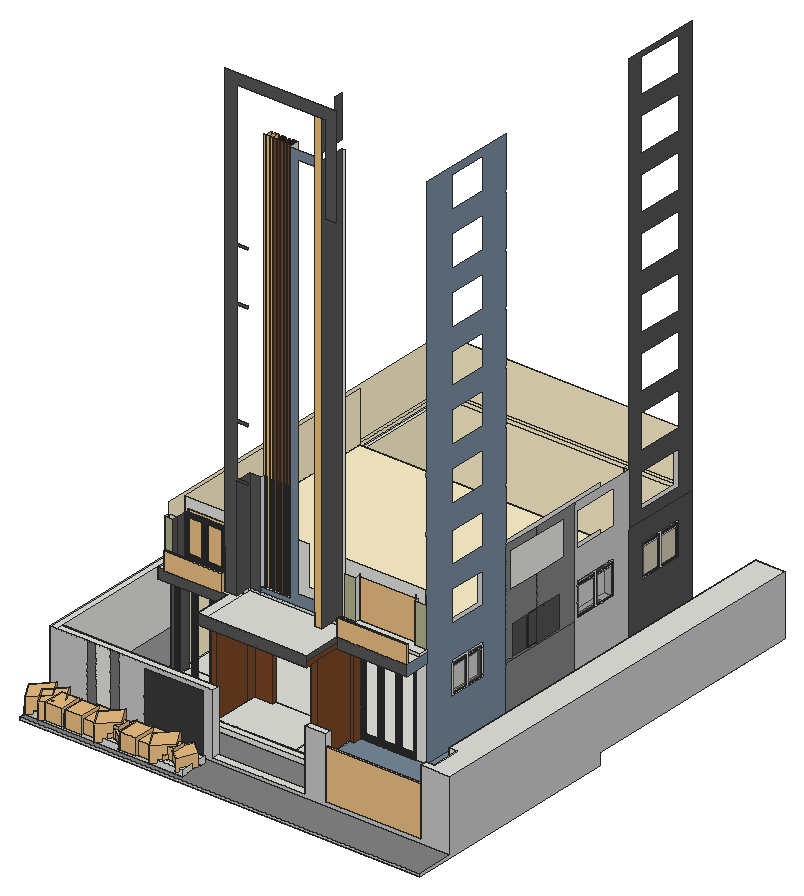
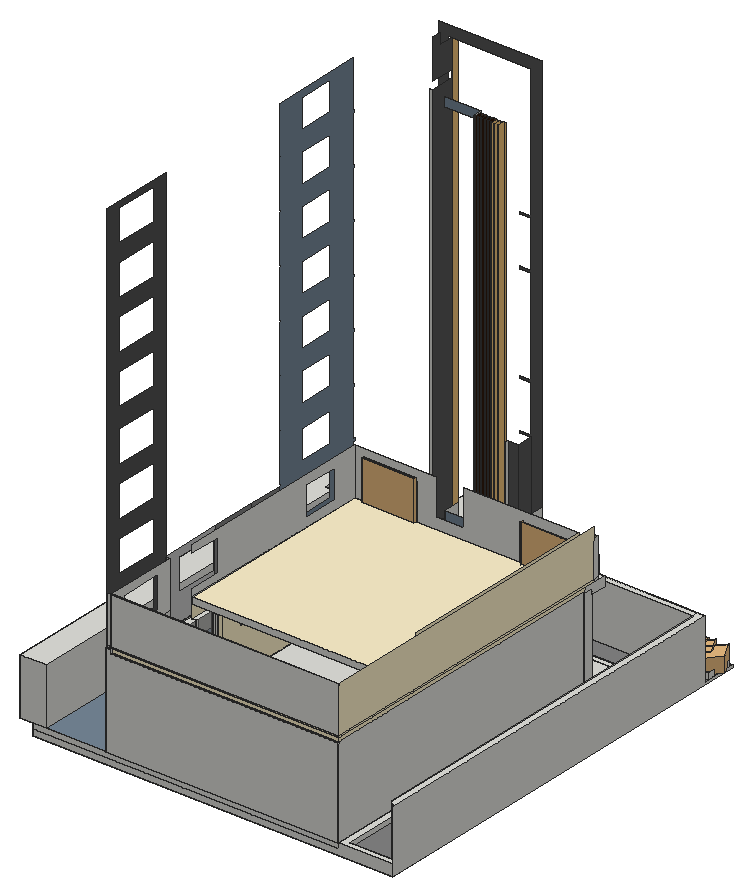
# SketchUp Ruby script. Lengths in inches.
U = 1.inch
M = Sketchup.active_model
def pt(a) = Geom::Point3d.new(a.map { |v| v * U })
def face(e, loops, mat)
  f = e.add_face(loops[0].map { |a| pt(a) })
  loops[1..].each { |l| e.add_face(l.map { |a| pt(a) }).erase! }
  f.material = f.back_material = mat if mat
  f
end
# faces: each face lists its corners as indices into pts; further lists are holes
def faces(e, pts, list, mat = nil) = list.each { |f| face(e, (f[0].is_a?(Array) ? f : [f]).map { |l| l.map { |i| pts[i] } }, mat) }
# xy, xz, yz: faces in a plane at the given z, y or x. An outline is a flat list of corners, or four numbers for a rectangle; further outlines are holes
def ring(l) = l.size == 4 ? [[l[0], l[1]], [l[2], l[1]], [l[2], l[3]], [l[0], l[3]]] : l.each_slice(2).to_a
def flat(e, list, mat, &to3) = list.each { |f| face(e, (f[0].is_a?(Array) ? f : [f]).map { |l| ring(l).map { |u, v| to3.(u, v) } }, mat) }
def xy(e, z, list, mat = nil) = flat(e, list, mat) { |x, y| [x, y, z] }
def xz(e, y, list, mat = nil) = flat(e, list, mat) { |x, z| [x, y, z] }
def yz(e, x, list, mat = nil) = flat(e, list, mat) { |y, z| [x, y, z] }
def lines(e, pts, list) = list.each { |a, b| e.add_line(pt(pts[a]), pt(pts[b])) }
# prism: a flat outline (further loops are holes) pulled along v
def prism(e, loops, v, mat = nil)
  f = face(e, loops, mat); d = Geom::Vector3d.new(v.map { |x| x * U })
  f.pushpull(f.normal.samedirection?(d) ? d.length : -d.length)
end
def box(e, o, s, mat = nil) = prism(e, [[o, [o[0] + s[0], o[1], o[2]], [o[0] + s[0], o[1] + s[1], o[2]], [o[0], o[1] + s[1], o[2]]]], [0, 0, s[2]], mat)
def at(x, y, z, deg = 0) = Geom::Transformation.translation(pt([x, y, z])) * Geom::Transformation.rotation(ORIGIN, Z_AXIS, deg.degrees)
def axes(o, x, y, z) = Geom::Transformation.new([*x, 0, *y, 0, *z, 0, *pt(o).to_a, 1])
def part(name) = M.definitions.add(name)
# library, detail: a bought-in or finely detailed component or shape, given as its bounding box
def library(name, o, s) = part(name).tap { |d| box(d.entities, o, s) }
def detail(e, o, s) = box(e.add_group.entities, o, s)
def put(e, d, t, mat = nil) = e.add_instance(d, t).tap { |i| i.material = mat if mat }
def group(e, t, mat = nil) = e.add_group.tap { |g| g.transformation = t; g.material = mat if mat }.entities
root = M.entities
M.materials.add("Material__1").color = [95, 70, 46]
M.materials.add("Wine2").color = [0, 0, 0]
M.materials["Wine2"].alpha = 0
M.materials.add("[0110_LightSlateGray]").color = [119, 136, 153]
M.materials.add("[0130_Gainsboro]").color = [39, 45, 50]
M.materials.add("[0133_Gray]").color = [128, 128, 128]
M.materials.add("[0135_DarkGray]1").color = [81, 81, 81]
M.materials.add("[Color D01]").color = [255, 242, 204]
M.materials.add("[Color E01]").color = [178, 178, 142]
M.materials.add("[Color M02]").color = [198, 198, 198]
M.materials.add("[Color M05]").color = [114, 114, 114]
M.materials.add("[Color M06]").color = [86, 86, 86]
M.materials.add("[Color M07]").color = [58, 58, 58]
M.materials.add("[Tile Grey]").color = [132, 132, 132]
M.materials.add("[Translucent Glass Gray]").color = [128, 128, 128]
M.materials["[Translucent Glass Gray]"].alpha = 0.5
M.materials.add("[Wood Bamboo]").color = [214, 127, 52]
M.materials.add("[Wood Cherry Original]").color = [48, 27, 13]
M.materials.add("[Wood OSB]").color = [240, 195, 122]
M.materials.add("[Wood Veneer 01]").color = [120, 70, 37]
c1 = library("Group\#74",[-84.69,-90.07,-0.36],[176.51,175.13,171.4])
c2 = library("Areca palm plant",[0,0,0],[49.1,36.6,54.46])
c3 = library("Group\#130",[-7.34,-1.2,0],[38.67,35.81,49.04])
c4 = library("Group20\#1",[-20.81,-17.08,3.79],[39.86,39.43,37.51])
c5 = library("Group38\#2",[14.01,28.44,-23.43],[18.58,18.32,38.89])
c6 = library("Slatted entrance gates",[-0.09,68.76,-0.1],[160,5.32,60.06])
c7 = part("Framed glazing panel")
xy(c7.entities,0,[[0,-0.98,43.07,0],[0,0,43.07,1.4]],"[0130_Gainsboro]")
xy(c7.entities,0.3,[[0.3,-1.43,42.77,-0.98]],"[0130_Gainsboro]")
xy(c7.entities,2.95,[[2.95,-1.43,40.12,-0.63],[2.95,-0.63,40.12,0],[2.95,0,40.12,0.64],[2.95,0.64,40.12,1.4]],"[0130_Gainsboro]")
xy(c7.entities,3.54,[[3.54,-0.63,39.53,0],[3.54,0,39.53,0.64]],"[0130_Gainsboro]")
xy(c7.entities,111.8125,[[3.54,-0.63,39.53,0],[3.54,0,39.53,0.64]],"[0130_Gainsboro]")
xy(c7.entities,112.4,[[2.95,-1.43,40.12,-0.63],[2.95,-0.63,40.12,0],[2.95,0,40.12,0.64],[2.95,0.64,40.12,1.4]],"[0130_Gainsboro]")
xy(c7.entities,115.05,[[0.3,-1.43,42.77,-0.98]],"[0130_Gainsboro]")
xy(c7.entities,115.35,[[0,-0.98,43.07,0],[0,0,43.07,1.4]],"[0130_Gainsboro]")
xz(c7.entities,-1.43,[[[0.3,0.3,42.77,115.05],[2.95,2.95,40.12,112.4]]],"[0130_Gainsboro]")
xz(c7.entities,-0.98,[[[0,0,43.07,115.35],[0.3,0.3,42.77,115.05]]],"[0130_Gainsboro]")
xz(c7.entities,-0.63,[[[2.95,2.95,40.12,112.4],[3.54,3.54,39.53,111.8125]]],"[0130_Gainsboro]")
xz(c7.entities,0,[[3.54,3.54,39.53,111.8125]],"Wine2")
xz(c7.entities,0,[[[0,0,43.07,115.35],[2.95,2.95,40.12,112.4]],[[2.95,2.95,40.12,112.4],[3.54,3.54,39.53,111.8125]]],"[0130_Gainsboro]")
xz(c7.entities,0.64,[[[2.95,2.95,40.12,112.4],[3.54,3.54,39.53,111.8125]]],"[0130_Gainsboro]")
xz(c7.entities,1.4,[[[0,0,43.07,115.35],[2.95,2.95,40.12,112.4]]],"[0130_Gainsboro]")
yz(c7.entities,0,[[-0.98,0,0,115.35],[0,0,1.4,115.35]],"[0130_Gainsboro]")
yz(c7.entities,0.3,[[-1.43,0.3,-0.98,115.05]],"[0130_Gainsboro]")
yz(c7.entities,2.95,[[-1.43,2.95,-0.63,112.4],[-0.63,2.95,0,112.4],[0,2.95,0.64,112.4],[0.64,2.95,1.4,112.4]],"[0130_Gainsboro]")
yz(c7.entities,3.54,[[-0.63,3.54,0,111.8125],[0,3.54,0.64,111.8125]],"[0130_Gainsboro]")
yz(c7.entities,39.53,[[-0.63,3.54,0,111.8125],[0,3.54,0.64,111.8125]],"[0130_Gainsboro]")
yz(c7.entities,40.12,[[-1.43,2.95,-0.63,112.4],[-0.63,2.95,0,112.4],[0,2.95,0.64,112.4],[0.64,2.95,1.4,112.4]],"[0130_Gainsboro]")
yz(c7.entities,42.77,[[-1.43,0.3,-0.98,115.05]],"[0130_Gainsboro]")
yz(c7.entities,43.07,[[-0.98,0,0,115.35],[0,0,1.4,115.35]],"[0130_Gainsboro]")
c8 = part("Glazing assembly")
put(c8.entities,c7,axes([90.57,1.43,0],[1.05148,0,0],[0,1,0],[0,0,1]))
put(c8.entities,c7,axes([0,1.43,0],[1.05148,0,0],[0,1,0],[0,0,1]))
put(c8.entities,c7,axes([45.29,1.43,0],[1.05148,0,0],[0,1,0],[0,0,1]))
c9 = part("Group\#3")
xy(c9.entities,0,[[0,0,32.48,1.97]])
xy(c9.entities,0.98,[[0.98,0,31.5,0.98],[0.98,0.98,31.5,1.97]])
xy(c9.entities,8.86,[[0.98,0,31.5,0.98],[0.98,0.98,31.5,1.97]])
xy(c9.entities,9.84,[[0,0,32.48,1.97]])
xz(c9.entities,0,[[[0,0,32.48,9.84],[0.98,0.98,31.5,8.86]]])
xz(c9.entities,0.98,[[0.98,0.98,31.5,8.86]],"[Translucent Glass Gray]")
xz(c9.entities,1.97,[[[0,0,32.48,9.84],[0.98,0.98,31.5,8.86]]])
yz(c9.entities,0,[[0,0,1.97,9.84]])
yz(c9.entities,0.98,[[0,0.98,0.98,8.86],[0.98,0.98,1.97,8.86]])
yz(c9.entities,31.5,[[0,0.98,0.98,8.86],[0.98,0.98,1.97,8.86]])
yz(c9.entities,32.48,[[0,0,1.97,9.84]])
c10 = part("Group\#4")
xy(c10.entities,0,[[0,0,32.48,1.97]])
xy(c10.entities,0.98,[[0.98,0,31.5,0.98],[0.98,0.98,31.5,1.97]])
xy(c10.entities,71.85,[[0.98,0,31.5,0.98],[0.98,0.98,31.5,1.97]])
xy(c10.entities,72.83,[[0,0,32.48,1.97]])
xz(c10.entities,0,[[[0,0,32.48,72.83],[0.98,0.98,31.5,71.85]]])
xz(c10.entities,0.98,[[0.98,0.98,31.5,71.85]],"[Translucent Glass Gray]")
xz(c10.entities,1.97,[[[0,0,32.48,72.83],[0.98,0.98,31.5,71.85]]])
yz(c10.entities,0,[[0,0,1.97,72.83]])
yz(c10.entities,0.98,[[0,0.98,0.98,71.85],[0.98,0.98,1.97,71.85]])
yz(c10.entities,31.5,[[0,0.98,0.98,71.85],[0.98,0.98,1.97,71.85]])
yz(c10.entities,32.48,[[0,0,1.97,72.83]])
c11 = part("FIXED+GLASS+WINDOW+WITH+TRANSOM")
g1 = group(c11.entities,at(0,0,0))
xy(g1,0,[[0,0,70.86,3.9375]])
xy(g1,1.97,[[1.97,0,34.45,0.98],[36.42,0,68.9,3.9375],[1.97,2.95,34.45,3.9375]])
xy(g1,86.61,[[1.97,0,34.45,3.9375],[34.45,0,36.42,3.9375],[36.42,0,68.9,3.9375]])
xy(g1,88.58,[[0,0,70.86,3.9375]])
xz(g1,0,[[[0,0,70.86,88.58],[1.97,1.97,34.45,86.61],[36.42,1.97,68.9,86.61]]])
xz(g1,3.9375,[[[0,0,70.86,88.58],[1.97,1.97,34.45,86.61],[36.42,1.97,68.9,86.61]]])
yz(g1,0,[[0,0,3.9375,88.58]])
yz(g1,1.97,[[0,1.97,3.9375,74.8],[0,76.77,3.9375,86.61]])
yz(g1,34.45,[[0,1.97,3.9375,86.61]])
yz(g1,36.42,[[0,1.97,3.9375,86.61]])
yz(g1,68.9,[[0,1.97,3.9375,86.61]])
yz(g1,70.86,[[0,0,3.9375,88.58]])
g2 = group(g1,at(1.97,0,74.8))
box(g2,[0,0,0],[66.93,3.9375,1.97])
put(g1,c9,at(1.97,0.98,76.77))
put(g1,c9,at(36.42,0.98,76.77))
put(g1,c10,at(1.97,0.98,1.97))
put(g1,c10,at(36.42,0.98,1.97))
c12 = library("Glass Railing",[0,0,0],[139.5,4.76,42])
c13 = library("Group5_1",[-7.56,-66.38,0.11],[6.33,135.04,120.95])
xy(root,-23.6875,[[0,0,0,1091.875,923.0625,1091.875,923.0625,537.75,956.9375,537.75,956.9375,0]])
xy(root,-17.4,[[0,0,956.9375,91]],"[Tile Grey]")
xy(root,-8,[[389.92,91,609.52,107.02],[658.23,91,886.57,107.02]])
xy(root,-8,[[16.02,107.02,907.04,107.02,907.04,173.85,121.35,173.85,121.35,1075.85,16.02,1075.85]],"[Tile Grey]")
xy(root,4.3125,[[121.35,173.85,886.57,173.85,886.57,189.875,137.375,189.875,137.375,1091.875,0,1091.875,16.02,1075.85,121.35,1075.85],[156.37,189.875,304.43,310.82],[363.41,189.875,507.41,310.82],[565.09,189.875,706.35,310.82]])
xy(root,5.625,[[547.97,185.5625,565.09,189.875],[137.375,189.875,156.37,280.75],[156.37,189.875,304.43,310.82],[304.43,189.875,304.43,310.82,363.41,310.82,363.41,301.625,320.43,301.625,320.43,189.875],[320.43,189.875,507.41,189.875,507.41,310.82,363.41,310.82,363.41,301.625,320.43,301.625],
  [507.41,189.875,547.97,301.625],[547.97,189.875,547.97,301.625,507.41,301.625,507.41,310.82,565.09,310.82,565.09,189.875],[565.09,279.375,575.47,310.82],[137.375,280.75,156.37,310.82],[706.35,301.625,733.4375,301.625,733.4375,1091.875,146.57,1091.875,146.57,832.49,721.74,832.49,721.74,310.82,706.35,310.82],
  [137.375,310.82,146.57,1091.875],[146.57,310.82,721.74,832.49],[733.4375,904.3,733.625,1091.875],[137.375,1091.875,733.4375,1094.4375]])
xy(root,5.625,[[565.09,189.875,886.57,189.875,886.57,1091.875,733.625,1091.875,733.625,904.3,733.4375,904.3,733.4375,301.625,706.35,301.625,706.35,310.82,575.47,310.82,575.47,279.375,565.09,279.375]],"[0110_LightSlateGray]")
xy(root,5.625,[[923.0625,537.75,956.9375,744.22],[923.0625,744.22,956.9375,904.3],[923.0625,904.3,956.9375,1091.875]],"[Color M02]")
xy(root,119.72,[[721.74,375.23,733.4375,467.6]])
xy(root,120.06,[[719.43,538.27,721.74,678.14]])
xy(root,120.52,[[711.11,750.25,721.74,832.49],[721.74,750.25,733.4375,750.25,733.4375,861.32,711.11,861.32,711.11,832.49,721.74,832.49],[733.4375,942.08,733.625,1053.14]])
xy(root,137,[[0,91,16.02,91,16.02,1075.85,0,1091.875],[16.02,91,389.92,107.02],[609.52,91,658.23,107.02]])
xy(root,150.625,[[886.57,91,956.9375,91,956.9375,1091.875,886.57,1091.875,886.57,173.85,907.04,173.85,907.04,107.02,886.57,107.02]])
xy(root,194.22,[[721.74,375.23,733.4375,467.6]])
xy(root,201.77,[[711.11,750.25,721.74,832.49],[721.74,750.25,721.74,832.49,711.11,832.49,711.11,861.32,733.4375,861.32,733.4375,750.25],[733.4375,942.08,733.625,1053.14]])
xy(root,202.93,[[719.43,538.27,721.74,678.14]])
xy(root,205.15,[[363.41,301.625,507.41,310.82]])
xy(root,220.35,[[304.43,151.125,304.43,189.875,320.43,189.875,320.43,279.375,547.97,279.375,547.97,185.5625,565.09,185.5625,565.09,151.125],[320.43,279.375,547.97,301.625]],"[Wood Bamboo]")
xy(root,220.77,[[137.375,240.3125,137.375,280.75,156.37,280.75,156.37,301.625,304.43,301.625,304.43,240.3125],[565.09,240.3125,565.09,279.375,575.47,279.375,575.47,301.625,733.4375,301.625,733.4375,240.3125]],"[Wood Bamboo]")
xy(root,233.58,[[156.37,301.625,304.43,310.82]])
xy(root,234.19,[[575.47,301.625,706.35,310.82]])
xy(root,236.5,[[137.375,310.82,146.57,1091.875],[137.375,1091.875,721.74,1094.4375]])
xy(root,245.625,[[304.43,151.125,326.68,261.5],[326.68,151.125,565.09,279.375],[137.375,240.3125,304.43,261.5],[565.09,240.3125,733.4375,279.375],[137.375,261.5,304.43,273.3125],
  [304.43,261.5,326.68,273.3125],[304.43,273.3125,326.68,279.375],[733.4375,904.3,733.625,1091.875],[721.74,1091.875,733.4375,1094.4375]])
xy(root,251.625,[[298.7,240.0625,326.68,261.5],[514.85,240.0625,529.32,279.375],[137.375,261.5,157.82,273.3125],[157.82,261.5,298.7,273.3125],[298.7,261.5,326.68,273.3125],
  [157.82,273.3125,298.7,310.82],[298.7,273.3125,298.7,310.82,563.32,310.82,563.32,301.625,529.32,301.625,529.32,279.375,326.68,279.375,326.68,273.3125],[529.32,279.375,536.21,301.625],[536.21,279.375,563.32,301.625],[563.32,279.375,563.32,310.82,704.2,310.82,704.2,301.625,733.4375,301.625,733.4375,279.375],
  [137.375,1091.875,721.74,1092.875]])
xy(root,251.625,[[146.57,310.82,721.74,832.49]],"[Color D01]")
xy(root,262.54,[[354.04,279.375,423.66,279.375,423.66,301.625,419.15,301.625,419.15,285.875,413.1,285.875,413.1,301.625,410.71,301.625,410.71,285.875,404.66,285.875,404.66,301.625,402.28,301.625,402.28,285.875,396.22,285.875,396.22,301.625,393.84,301.625,393.84,285.875,387.79,285.875,387.79,301.625,385.4,301.625,385.4,285.875,379.35,285.875,379.35,301.625,376.96,301.625,376.96,285.875,370.91,285.875,370.91,301.625,368.53,301.625,368.53,285.875,362.47,285.875,362.47,301.625,360.09,301.625,360.09,285.875,354.04,285.875]])
xz(root,0,[[0,-23.6875,956.9375,-17.4]],"[Color M02]")
xz(root,91,[[107.87,-17.4,141.375,137]])
xz(root,91,[[0,-17.4,87.26,137],[162.87,-17.4,223.1,-17.4,223.1,126.22,366.73,126.22,366.73,-17.4,956.9375,-17.4,956.9375,150.625,886.57,150.625,886.57,-8,658.23,-8,658.23,137,609.52,137,609.52,-8,389.92,-8,389.92,137,162.87,137]],"[Color M02]")
xz(root,91,[[87.26,-17.4,107.87,137],[141.375,-17.4,162.87,137]],"[Color M05]")
xz(root,91,[[223.1,-17.4,366.73,126.22]],"[Color M07]")
xz(root,107.02,[[16.02,-8,389.92,137],[609.52,-8,658.23,137],[886.57,-8,907.04,150.625]])
xz(root,151.125,[[304.43,220.35,565.09,245.625]],"[Color M06]")
xz(root,173.85,[[121.35,-8,156.37,4.3125],[156.37,-8,886.57,4.3125],[886.57,-8,907.04,150.625]])
xz(root,185.5625,[[547.97,5.625,565.09,220.35]],"[Wood Veneer 01]")
xz(root,189.875,[[137.375,4.3125,156.37,5.625],[156.37,4.3125,304.43,5.625],[304.43,4.3125,363.41,5.625],[363.41,4.3125,507.41,5.625],[507.41,4.3125,565.09,5.625],
  [565.09,4.3125,706.35,5.625],[706.35,4.3125,886.57,5.625]])
xz(root,189.875,[[304.43,5.625,320.43,220.35]],"[Wood Veneer 01]")
xz(root,240.0625,[[298.7,251.625,326.68,251.625,326.68,497.625,354.04,497.625,354.04,503.625,326.68,503.625,326.68,623.625,354.04,623.625,354.04,629.625,326.68,629.625,326.68,875.625,354.04,875.625,354.04,881.625,326.68,881.625,326.68,1001.625,354.04,1001.625,354.04,1007.625,326.68,1007.625,326.68,1345.48,539.29,1345.48,539.29,1133.625,563.32,1133.625,563.32,1373.625,298.7,1373.625]],"[Color M06]")
xz(root,240.0625,[[514.85,251.625,529.32,1345.48]],"[Wood OSB]")
xz(root,240.3125,[[137.375,220.77,304.43,245.625],[565.09,220.77,733.4375,245.625]],"[Color M06]")
xz(root,261.5,[[137.375,245.625,326.68,251.625]])
xz(root,261.5,[[137.375,251.625,157.82,345.6875]],"[Color E01]")
xz(root,273.3125,[[137.375,245.625,326.68,251.625],[137.375,251.625,157.82,345.6875]])
xz(root,279.375,[[326.68,245.625,354.04,251.625],[354.04,245.625,733.4375,251.625]])
xz(root,279.375,[[354.04,251.625,514.85,251.625,514.85,279.6,442.42,279.6,442.42,1208.73,514.85,1208.73,514.85,1230.97,423.66,1230.97,423.66,262.54,354.04,262.54]],"[0110_LightSlateGray]")
xz(root,279.375,[[326.68,251.625,354.04,497.625]],"[Color M06]")
xz(root,279.375,[[565.09,5.625,575.47,220.77]],"[Wood Veneer 01]")
xz(root,280.75,[[137.375,5.625,156.37,220.77]],"[Color M06]")
xz(root,285.875,[[354.04,262.54,360.09,1230.97],[362.47,262.54,368.53,1230.97],[370.91,262.54,376.96,1230.97]],"[Wood OSB]")
xz(root,285.875,[[379.35,262.54,385.4,1230.97],[387.79,262.54,393.84,1230.97],[396.22,262.54,402.28,1230.97],[404.66,262.54,410.71,1230.97],[413.1,262.54,419.15,1230.97]],"[Wood Veneer 01]")
xz(root,301.625,[[706.35,5.625,733.4375,220.77],[156.37,220.77,304.43,233.58],[575.47,220.77,706.35,234.19],[704.2,236.5,733.4375,245.625],[704.2,245.625,733.4375,251.625],
  [529.32,251.625,536.21,1253.625],[360.09,262.54,362.47,1230.97],[368.53,262.54,370.91,1230.97],[376.96,262.54,379.35,1230.97]])
xz(root,301.625,[[536.21,251.625,563.32,345.6875],[704.2,251.625,733.4375,345.6875]],"[Color E01]")
xz(root,301.625,[[385.4,262.54,387.79,1230.97],[393.84,262.54,396.22,1230.97],[402.28,262.54,404.66,1230.97],[410.71,262.54,413.1,1230.97],[419.15,262.54,423.66,1230.97]],"[Wood Cherry Original]")
xz(root,301.625,[[320.43,5.625,363.41,5.625,363.41,205.15,507.41,205.15,507.41,5.625,547.97,5.625,547.97,220.35,320.43,220.35]],"[Wood Veneer 01]")
xz(root,310.82,[[146.57,-8,156.37,5.625],[706.35,-8,721.74,5.625],[156.37,4.3125,304.43,5.625],[363.41,4.3125,507.41,5.625],[565.09,4.3125,706.35,5.625],
  [137.375,5.625,146.57,236.5],[146.57,5.625,146.57,236.5,157.82,236.5,157.82,245.625,704.2,245.625,704.2,236.5,721.74,236.5,721.74,5.625,706.35,5.625,706.35,234.19,575.47,234.19,575.47,5.625,507.41,5.625,507.41,205.15,363.41,205.15,363.41,5.625,304.43,5.625,304.43,233.58,156.37,233.58,156.37,5.625],[146.57,236.5,157.82,245.625],[704.2,236.5,721.74,245.625],[146.57,245.625,157.82,251.625],
  [704.2,245.625,721.74,251.625],[146.57,251.625,146.57,371.625,442.42,371.625,442.42,279.6,514.85,279.6,514.85,371.625,721.74,371.625,721.74,251.625,704.2,251.625,704.2,345.6875,563.32,345.6875,563.32,251.625,298.7,251.625,298.7,345.6875,157.82,345.6875,157.82,251.625]])
xz(root,375.23,[[721.74,119.72,733.4375,194.22]])
xz(root,467.6,[[721.74,119.72,733.4375,194.22]],"[Color D01]")
xz(root,537.75,[[923.0625,-23.6875,956.9375,5.625]],"[Color M02]")
xz(root,538.27,[[719.43,120.06,721.74,202.93]])
xz(root,678.14,[[719.43,120.06,721.74,202.93]])
xz(root,750.25,[[721.74,120.52,733.4375,201.77]])
xz(root,750.25,[[711.11,120.52,721.74,201.77]],"[Color D01]")
xz(root,832.49,[[146.57,-8,721.74,5.625],[146.57,236.5,721.74,251.625]])
xz(root,861.32,[[711.11,120.52,733.4375,201.77]])
xz(root,904.3,[[733.4375,5.625,733.625,236.5],[721.74,236.5,733.4375,251.625],[733.4375,236.5,733.625,245.625],[721.74,251.625,733.4375,371.625]])
xz(root,942.08,[[733.4375,120.52,733.625,201.77]])
xz(root,1053.14,[[733.4375,120.52,733.625,201.77]])
xz(root,1075.85,[[16.02,-8,121.35,4.3125]])
xz(root,1091.875,[[0,-23.6875,0,4.3125,137.375,4.3125,137.375,-8,923.0625,-8,923.0625,-23.6875],[137.375,-8,923.0625,5.625],[733.4375,5.625,733.625,245.625],[886.57,5.625,956.9375,150.625],[721.74,245.625,733.4375,251.625],
  [721.74,251.625,733.4375,371.625]])
xz(root,1091.875,[[146.57,5.625,733.4375,5.625,733.4375,245.625,721.74,245.625,721.74,236.5,146.57,236.5],[137.375,236.5,721.74,245.625],[137.375,245.625,721.74,251.625],[137.375,251.625,721.74,371.625]],"[Color D01]")
xz(root,1092.875,[[137.375,251.625,721.74,371.625]])
xz(root,1094.4375,[[137.375,5.625,137.375,236.5,721.74,236.5,721.74,245.625,733.4375,245.625,733.4375,5.625]])
yz(root,0,[[0,-23.6875,0,-17.4,91,-17.4,91,137,1091.875,137,1091.875,-23.6875]])
yz(root,16.02,[[107.02,-8,1075.85,137]])
yz(root,121.35,[[173.85,-8,1075.85,4.3125]])
yz(root,137.375,[[189.875,4.3125,1091.875,5.625],[280.75,5.625,301.625,233.58],[310.82,5.625,1091.875,236.5],[1091.875,5.625,1094.4375,236.5],[240.3125,220.77,240.3125,245.625,301.625,245.625,301.625,233.58,280.75,233.58,280.75,220.77],
  [261.5,245.625,273.3125,251.625],[261.5,251.625,273.3125,345.6875],[1091.875,251.625,1092.875,371.625]])
yz(root,137.375,[[301.625,236.5,1091.875,245.625],[273.3125,245.625,1091.875,251.625],[273.3125,251.625,1091.875,371.625]],"[Color D01]")
yz(root,146.57,[[310.82,-8,832.49,5.625],[310.82,245.625,832.49,251.625]])
yz(root,146.57,[[310.82,5.625,1091.875,236.5],[310.82,236.5,832.49,245.625],[310.82,251.625,832.49,371.625]],"[Color D01]")
yz(root,156.37,[[189.875,4.3125,280.75,5.625],[280.75,4.3125,310.82,5.625]])
yz(root,156.37,[[280.75,5.625,310.82,5.625,310.82,233.58,301.625,233.58,301.625,220.77,280.75,220.77]],"[Color M06]")
yz(root,157.82,[[261.5,251.625,273.3125,345.6875],[273.3125,251.625,310.82,345.6875]],"[Color M06]")
yz(root,298.7,[[240.0625,251.625,310.82,345.6875]])
yz(root,304.43,[[189.875,4.3125,279.375,5.625],[279.375,4.3125,310.82,5.625]])
yz(root,304.43,[[189.875,5.625,189.875,220.35,151.125,220.35,151.125,233.58,240.3125,233.58,240.3125,220.77,279.375,220.77,279.375,5.625],[279.375,5.625,279.375,220.77,301.625,220.77,301.625,233.58,310.82,233.58,310.82,5.625],[151.125,233.58,240.3125,245.625]],"[Wood Veneer 01]")
yz(root,320.43,[[189.875,5.625,279.375,220.35],[279.375,5.625,301.625,220.35]],"[Wood Veneer 01]")
yz(root,326.68,[[261.5,245.625,273.3125,251.625],[273.3125,245.625,279.375,251.625]])
yz(root,326.68,[[240.0625,251.625,279.375,497.625]],"[Color M06]")
yz(root,354.04,[[279.375,262.54,285.875,497.625]])
yz(root,360.09,[[285.875,262.54,301.625,1230.97]],"[Wood OSB]")
yz(root,362.47,[[285.875,262.54,301.625,497.625]])
yz(root,363.41,[[301.625,4.3125,310.82,5.625]])
yz(root,363.41,[[301.625,5.625,310.82,205.15]],"[Wood Veneer 01]")
yz(root,368.53,[[285.875,262.54,301.625,1230.97]],"[Wood OSB]")
yz(root,370.91,[[285.875,262.54,301.625,497.625]])
yz(root,376.96,[[285.875,262.54,301.625,1230.97]],"[Wood OSB]")
yz(root,379.35,[[285.875,262.54,301.625,497.625]])
yz(root,385.4,[[285.875,262.54,301.625,1230.97]],"[Wood Cherry Original]")
yz(root,387.79,[[285.875,262.54,301.625,497.625]])
yz(root,389.92,[[91,-8,107.02,137]])
yz(root,393.84,[[285.875,262.54,301.625,1230.97]],"[Wood Cherry Original]")
yz(root,396.22,[[285.875,262.54,301.625,497.625]])
yz(root,402.28,[[285.875,262.54,301.625,1230.97]],"[Wood Cherry Original]")
yz(root,404.66,[[285.875,262.54,301.625,497.625]])
yz(root,410.71,[[285.875,262.54,301.625,1230.97]],"[Wood Cherry Original]")
yz(root,413.1,[[285.875,262.54,301.625,497.625]])
yz(root,419.15,[[285.875,262.54,301.625,1230.97]],"[Wood Cherry Original]")
yz(root,423.66,[[279.375,262.54,301.625,1230.97]])
yz(root,507.41,[[189.875,4.3125,301.625,5.625],[301.625,4.3125,310.82,5.625],[301.625,5.625,310.82,205.15]])
yz(root,514.85,[[240.0625,251.625,279.375,279.6]])
yz(root,529.32,[[240.0625,251.625,301.625,251.625,301.625,1253.625,240.3125,1253.625,240.3125,1272.5,301.625,1272.5,301.625,1373.625,279.375,1373.625,279.375,1345.48,240.0625,1345.48]],"[Color M06]")
yz(root,547.97,[[185.5625,5.625,279.375,220.35],[279.375,5.625,301.625,220.35]],"[Wood Veneer 01]")
yz(root,563.32,[[301.625,251.625,310.82,345.6875]])
yz(root,565.09,[[189.875,4.3125,279.375,5.625],[279.375,4.3125,310.82,5.625]])
yz(root,565.09,[[151.125,234.19,240.3125,245.625]],"[Color M06]")
yz(root,565.09,[[185.5625,5.625,279.375,5.625,279.375,220.77,240.3125,220.77,185.5625,220.35],[151.125,220.35,185.5625,220.35,240.3125,220.77,240.3125,234.19,151.125,234.19]],"[Wood Veneer 01]")
yz(root,575.47,[[279.375,5.625,310.82,5.625,310.82,234.19,301.625,234.19,301.625,220.77,279.375,220.77]],"[Wood Veneer 01]")
yz(root,609.52,[[91,-8,107.02,137]])
yz(root,658.23,[[91,-8,107.02,137]])
yz(root,704.2,[[301.625,236.5,310.82,251.625],[301.625,251.625,310.82,345.6875]])
yz(root,706.35,[[301.625,4.3125,310.82,5.625],[301.625,5.625,310.82,234.19]])
yz(root,719.43,[[538.27,120.06,678.14,202.93]],"[Color D01]")
yz(root,721.74,[[310.82,-8,832.49,5.625],[538.27,120.06,678.14,202.93],[310.82,236.5,832.49,245.625],[904.3,236.5,1091.875,251.625],[1091.875,236.5,1094.4375,245.625],
  [310.82,245.625,832.49,251.625],[[310.82,251.625,310.82,371.625,832.49,371.625,832.49,352.63,750.25,352.63,750.25,271.38,832.49,271.38,832.49,251.625],[375.23,274.03,467.6,348.53]],[[904.3,251.625,1091.875,371.625],[942.08,270.83,1053.14,352.08]],[1091.875,251.625,1092.875,371.625]])
yz(root,721.74,[[[310.82,5.625,310.82,236.5,832.49,236.5,832.49,201.77,750.25,201.77,750.25,120.52,832.49,120.52,832.49,5.625],[538.27,120.06,678.14,202.93],[375.23,119.72,467.6,194.22]]],"[Color D01]")
yz(root,733.4375,[[[904.3,5.625,1091.875,245.625],[942.08,120.52,1053.14,201.77]],[1091.875,5.625,1094.4375,245.625],[279.375,245.625,301.625,251.625]])
yz(root,733.4375,[[[301.625,5.625,537.75,5.625,537.75,371.625,534.42,371.625,534.42,377.625,537.75,377.625,537.75,497.625,534.42,497.625,534.42,503.625,537.75,503.625,537.75,623.625,534.42,623.625,534.42,629.625,537.75,629.625,537.75,749.625,534.42,749.625,534.42,755.625,537.75,755.625,537.75,875.625,534.42,875.625,534.42,881.625,537.75,881.625,537.75,1001.625,534.42,1001.625,534.42,1007.625,537.75,1007.625,537.75,1127.625,534.42,1127.625,534.42,1133.625,537.75,1133.625,537.75,1253.625,301.625,1253.625,301.625,1133.625,300.15,1133.625,300.15,1127.625,301.625,1127.625,301.625,1007.625,300.15,1007.625,300.15,1001.625,301.625,1001.625,301.625,881.625,300.15,881.625,300.15,875.625,301.625,875.625,301.625,755.625,300.15,755.625,300.15,749.625,301.625,749.625,301.625,629.625,298.875,629.625,298.875,623.625,301.625,623.625,301.625,503.625,298.875,503.625,298.875,497.625,301.625,497.625,301.625,377.625,297.25,377.625,297.25,371.625,301.625,371.625],[375.23,119.72,467.6,194.22],[375.23,274.03,467.6,348.53],[375.23,400.03,467.6,474.53],[375.23,532.03,467.6,606.53],[375.23,784.03,467.6,858.53],[375.23,658.03,467.6,732.53],[375.23,910.03,467.6,984.53],[375.23,1162.03,467.6,1236.53],[375.23,1036.03,467.6,1110.53]],[240.3125,220.77,301.625,245.625]],"[0110_LightSlateGray]")
yz(root,733.4375,[[537.75,5.625,744.22,116.83],[537.75,116.83,744.22,116.83,744.22,371.625,628.83,371.625,628.83,353.62,709.1,353.62,709.1,270.75,628.83,270.75,628.83,196.39,694.625,196.39,694.625,122.83,537.75,122.83],[537.75,122.83,553.875,122.83,553.875,196.39,628.83,196.39,628.83,270.75,549.1,270.75,549.1,353.62,628.83,353.62,628.83,371.625,537.75,371.625]],"[0133_Gray]")
yz(root,733.4375,[[553.875,122.83,628.83,196.39],[628.83,122.83,694.625,196.39],[[904.3,245.625,1091.875,1253.625],[942.08,270.83,1053.14,352.08],[942.08,396.83,1053.14,478.08],[942.08,522.83,1053.14,604.08],[942.08,648.83,1053.14,730.08],[942.08,780.83,1053.14,862.08],[942.08,906.83,1053.14,988.08],[942.08,1032.83,1053.14,1114.08],[942.08,1158.83,1053.14,1240.08]]],"[0135_DarkGray]1")
yz(root,733.4375,[[[744.22,5.625,904.3,371.625],[750.25,120.52,861.32,201.77],[750.25,271.38,861.32,352.63]]],"[Color M02]")
yz(root,733.625,[[[904.3,5.625,1091.875,245.625],[942.08,120.52,1053.14,201.77]]],"[0135_DarkGray]1")
yz(root,886.57,[[91,-8,107.02,150.625],[173.85,4.3125,173.85,150.625,1091.875,150.625,1091.875,5.625,189.875,5.625,189.875,4.3125]])
yz(root,907.04,[[107.02,-8,173.85,150.625]])
yz(root,923.0625,[[537.75,-23.6875,744.22,5.625]],"[0133_Gray]")
yz(root,923.0625,[[904.3,-23.6875,1091.875,5.625]],"[0135_DarkGray]1")
yz(root,923.0625,[[744.22,-23.6875,904.3,5.625]],"[Color M02]")
yz(root,956.9375,[[0,-23.6875,537.75,-23.6875,537.75,5.625,1091.875,5.625,1091.875,150.625,91,150.625,91,-17.4,0,-17.4]],"[Color M02]")
p = [[16.02,1075.85,4.3125],[0,1091.875,4.3125],[0,1091.875,137],[16.02,1075.85,137],[157.82,301.625,236.5],[157.82,310.82,236.5],
  [156.37,310.82,-8],[156.37,189.875,-8]]
faces(root,p,[[0,1,2,3]])
lines(root,p,[[4,5],[6,7]])
g3 = group(root,at(380.73,12.2,-17.4))
xy(g3,0,[[-380.73,0,0,10.74],[-380.73,53.7,0,64.44]])
xy(g3,3,[[-380.73,10.74,0,53.7]])
xy(g3,7,[[-372.62,10.74,-8.11,53.7]],"Material__1")
xy(g3,15,[[[-380.73,0,0,64.44],[-372.62,10.74,-8.11,53.7]]])
xz(g3,0,[[-380.73,0,0,15]])
xz(g3,10.74,[[-380.73,0,0,3],[-372.62,7,-8.11,15]])
xz(g3,53.7,[[-380.73,0,0,3],[-372.62,7,-8.11,15]])
xz(g3,64.44,[[-380.73,0,0,15]])
yz(g3,-380.73,[[0,0,0,15,64.44,15,64.44,0,53.7,0,53.7,3,10.74,3,10.74,0]])
yz(g3,-372.62,[[10.74,7,53.7,15]])
yz(g3,-8.11,[[10.74,7,53.7,15]])
yz(g3,0,[[0,0,10.74,0,10.74,3,53.7,3,53.7,0,64.44,0,64.44,15,0,15]])
put(root,c1,axes([157.41,38.93,-11.35],[0.11085,-0.0888,0],[0.064,0.15381,0],[0,0,0.10522]))
put(root,c1,axes([131.53,38.93,-11.35],[0.11085,-0.0888,0],[0.064,0.15381,0],[0,0,0.10522]))
put(root,c1,axes([192.5625,38.93,-11.35],[0.11085,-0.0888,0],[0.064,0.15381,0],[0,0,0.10522]))
put(root,c1,axes([323.9,38.93,-11.35],[0.11085,-0.0888,0],[0.064,0.15381,0],[0,0,0.10522]))
put(root,c1,axes([288.75,38.93,-11.35],[0.11085,-0.0888,0],[0.064,0.15381,0],[0,0,0.10522]))
put(root,c1,axes([262.87,38.93,-11.35],[0.11085,-0.0888,0],[0.064,0.15381,0],[0,0,0.10522]))
put(root,c1,axes([224.34,42.98,-11.33],[0.18172,-0.14558,0],[0.10491,0.25215,0],[0,0,0.1725]))
put(root,c1,axes([360.36,42.98,-11.33],[0.18172,-0.14558,0],[0.10491,0.25215,0],[0,0,0.1725]))
put(root,c1,axes([93,42.98,-11.33],[0.18172,-0.14558,0],[0.10491,0.25215,0],[0,0,0.1725]))
put(root,c2,axes([176.38,1.11,-11.32],[0.72486,0.80581,0],[-0.68351,1.18385,0],[0,0,0.72]))
put(root,c2,axes([307.72,1.11,-11.32],[0.72486,0.80581,0],[-0.68351,1.18385,0],[0,0,0.72]))
put(root,c2,axes([42.88,1.11,-11.32],[0.72486,0.80581,0],[-0.68351,1.18385,0],[0,0,0.72]))
put(root,c2,axes([10.38,1.11,-11.32],[0.72486,0.80581,0],[-0.68351,1.18385,0],[0,0,0.72]))
put(root,c3,axes([264.75,56.84,-9.4],[-1.0191,0,0],[0,-1.4141,0],[0,0,0.79]))
put(root,c3,axes([133.41,56.84,-9.4],[-1.0191,0,0],[0,-1.4141,0],[0,0,0.79]))
put(root,c3,axes([86.25,56.84,-9.4],[-1.0191,0,0],[0,-1.4141,0],[0,0,0.79]))
put(root,c4,axes([277.5625,46.16,-12.625],[-1.0965,0,0],[0,-1.5215,0],[0,0,0.85]))
put(root,c4,axes([146.22,46.16,-12.625],[-1.0965,0,0],[0,-1.5215,0],[0,0,0.85]))
put(root,c5,axes([382.22,4.86,10.77],[0,1.58379,0],[-1.22129,0,0],[0,0,0.85826]))
put(root,c5,axes([250.88,4.86,10.77],[0,1.58379,0],[-1.22129,0,0],[0,0,0.85826]))
put(root,c6,axes([658.36,-5.94,-7.81],[1.4241,0,0],[0,1.41,0],[0,0,1.9458]))
put(root,c8,axes([156.37,280.75,5.625],[0.94751,0,0],[0,-4,0],[0,0,1.86508]))
put(root,c8,axes([575.47,312.95,5.625],[0.94751,0,0],[0,-4,0],[0,0,1.86508]))
put(root,c11,axes([733.4375,375.23,119.72],[0,1.30355,0],[-1,0,0],[0,0,0.84102]))
put(root,c11,axes([733.4375,750.25,120.52],[0,1.56726,0],[-1,0,0],[0,0,0.91722]))
put(root,c11,axes([733.625,942.08,120.52],[0,1.56726,0],[-1,0,0],[0,0,0.91722]))
put(root,c8,axes([733.4375,553.875,122.83],[0,1.03599,0],[-1,0,0],[0,0,0.63771]))
put(root,c12,at(154.24,238.3,245.625))
put(root,c12,axes([566.04,240.3125,245.625],[1.2,0,0],[0,1,0],[0,0,1]))
put(root,c13,axes([222.85,306.6875,246.9375],[0,-1,0],[1,0,0],[0,0,0.83156]))
put(root,c8,axes([157.82,303.39,251.625],[1.03691,0,0],[0,-4,0],[0,0,0.80657]))
put(root,c13,axes([630.79,309.6,251.54],[0,-1,0],[1,0,0],[0,0,0.83156]))
